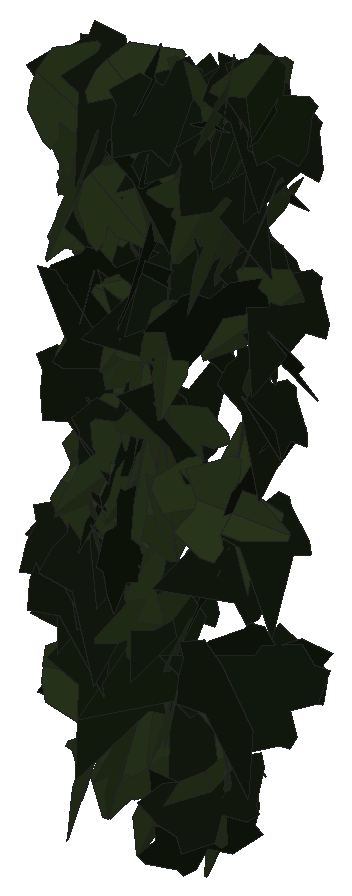
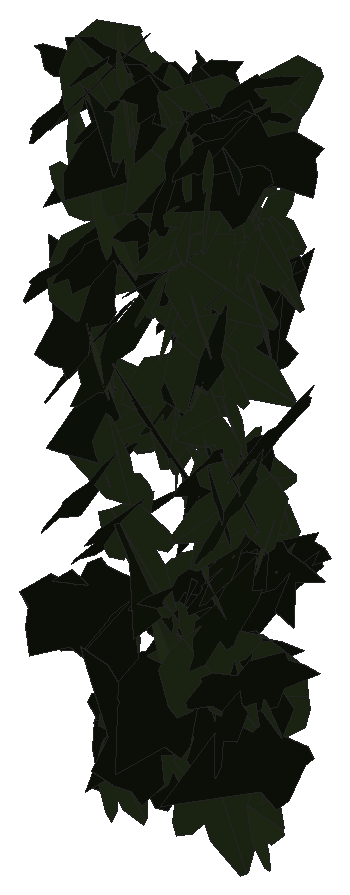
# SketchUp Ruby script. Lengths in inches.
U = 1.inch
M = Sketchup.active_model
def pt(a) = Geom::Point3d.new(a.map { |v| v * U })
def face(e, loops, mat)
  f = e.add_face(loops[0].map { |a| pt(a) })
  loops[1..].each { |l| e.add_face(l.map { |a| pt(a) }).erase! }
  f.material = f.back_material = mat if mat
  f
end
# faces: each face lists its corners as indices into pts; further lists are holes
def faces(e, pts, list, mat = nil) = list.each { |f| face(e, (f[0].is_a?(Array) ? f : [f]).map { |l| l.map { |i| pts[i] } }, mat) }
# xy, xz, yz: faces in a plane at the given z, y or x. An outline is a flat list of corners, or four numbers for a rectangle; further outlines are holes
def ring(l) = l.size == 4 ? [[l[0], l[1]], [l[2], l[1]], [l[2], l[3]], [l[0], l[3]]] : l.each_slice(2).to_a
def flat(e, list, mat, &to3) = list.each { |f| face(e, (f[0].is_a?(Array) ? f : [f]).map { |l| ring(l).map { |u, v| to3.(u, v) } }, mat) }
def xy(e, z, list, mat = nil) = flat(e, list, mat) { |x, y| [x, y, z] }
def xz(e, y, list, mat = nil) = flat(e, list, mat) { |x, z| [x, y, z] }
def yz(e, x, list, mat = nil) = flat(e, list, mat) { |y, z| [x, y, z] }
def lines(e, pts, list) = list.each { |a, b| e.add_line(pt(pts[a]), pt(pts[b])) }
# prism: a flat outline (further loops are holes) pulled along v
def prism(e, loops, v, mat = nil)
  f = face(e, loops, mat); d = Geom::Vector3d.new(v.map { |x| x * U })
  f.pushpull(f.normal.samedirection?(d) ? d.length : -d.length)
end
def box(e, o, s, mat = nil) = prism(e, [[o, [o[0] + s[0], o[1], o[2]], [o[0] + s[0], o[1] + s[1], o[2]], [o[0], o[1] + s[1], o[2]]]], [0, 0, s[2]], mat)
def at(x, y, z, deg = 0) = Geom::Transformation.translation(pt([x, y, z])) * Geom::Transformation.rotation(ORIGIN, Z_AXIS, deg.degrees)
def axes(o, x, y, z) = Geom::Transformation.new([*x, 0, *y, 0, *z, 0, *pt(o).to_a, 1])
def part(name) = M.definitions.add(name)
# library, detail: a bought-in or finely detailed component or shape, given as its bounding box
def library(name, o, s) = part(name).tap { |d| box(d.entities, o, s) }
def detail(e, o, s) = box(e.add_group.entities, o, s)
def put(e, d, t, mat = nil) = e.add_instance(d, t).tap { |i| i.material = mat if mat }
def group(e, t, mat = nil) = e.add_group.tap { |g| g.transformation = t; g.material = mat if mat }.entities
root = M.entities
M.materials.add("efeu1").color = [18, 25, 13]
M.materials.add("efeu2").color = [43, 57, 29]
c1 = part("ivyleaf_10")
p = [[0,0.5,-0.03],[-0.0625,2.02,-0.43],[-0.19,2.01,-0.46],[-0.54,1.05,-0.29],[-0.52,0.625,-0.18],[-0.83,0.76,-0.28],
  [-1.16,0.64,-0.33],[-1.15,0.33,-0.24],[-0.77,-0.39,0.02],[-0.3,-0.51,0.16],[0.04,-0.48,0.23],[-0.02,2.01,-0.4375],
  [-0.06,2.01,-0.43],[0.04,-0.49,0.23],[0.67,-0.49,0.14],[1.38,0.36,-0.2],[1.375,0.51,-0.24],[0.81,0.65,-0.19],
  [0.62,0.59,-0.15],[0.6,1.09,-0.28],[0.5,1.23,-0.31]]
faces(c1.entities,p,[[0,1,2,3,4,5,6,7,8,9,10],[11,12,0,13,14,15,16,17,18,19,20]],"efeu2")
c2 = part("ivyleaf_9")
p = [[1.54,2.16,1.25],[1.36,2.04,1.19],[-0.21,0.99,0.68],[-0.71,1.11,0.82],[-0.85,0.86,0.67],[-0.8,0.17,0.21],
  [-0.9,-0.01,0.1],[-0.67,-0.16,-0.02],[-0.08,-0.08,-0.05],[-0.03,-0.6,-0.4],[0.65,-0.88,-0.66],[0.83,-0.6,-0.49],
  [1.29,-0.42,-0.43],[1.8125,-0.07,-0.26],[1.21,0.44,0.15]]
faces(c2.entities,p,[[0,1,2,3,4,5,6,7,8,9,10,11,12,13,14]],"efeu1")
put(root,c1,axes([27.62,223.03,222.28],[-0.11697,0.34402,0.34346],[-0.14609,0.31206,-0.36232],[-0.46365,-0.18512,0.02751]))
put(root,c1,axes([27.55,223.54,221.27],[0.03739,0.32333,-0.37955],[-0.06683,-0.37393,-0.32513],[-0.4941,0.07505,0.01526]))
put(root,c2,axes([27.52,223.98,215.93],[-0.21987,-0.44229,-0.07768],[0.02759,0.07302,-0.49387],[0.44821,-0.22146,-0.0077]))
put(root,c2,axes([27.39,223.53,218.86],[0.19306,-0.44712,-0.11317],[-0.0519,0.10084,-0.48697],[0.45829,0.19978,-0.00747]))
put(root,c2,axes([27.375,223.71,222.54],[-0.12128,-0.22527,-0.42959],[0.20632,0.37681,-0.25583],[0.43901,-0.23932,0.00156]))
put(root,c1,axes([27.28,223.71,221.07],[0.31819,-0.13145,-0.3626],[0.33005,-0.15042,0.34416],[-0.19956,-0.45836,-0.00895]))
put(root,c2,axes([27.39,223.49,215.01],[0.39095,0.21573,0.22498],[0.19849,0.10596,-0.44651],[-0.24033,0.43845,-0.00279]))
put(root,c1,axes([27.84,223.37,221.11],[0.34552,-0.1496,-0.32899],[-0.30547,0.12234,-0.37646],[0.19313,0.46114,-0.00686]))
put(root,c1,axes([27.52,223.64,214.11],[0.14054,-0.2724,0.39503],[0.22811,-0.32421,-0.30472],[0.42215,0.26587,0.03314]))
put(root,c1,axes([27.64,222.8125,222.76],[-0.005,0.38256,0.3219],[-0.00797,0.32182,-0.38258],[-0.49991,-0.00896,0.00287]))
put(root,c1,axes([27.61,223.36,217.67],[-0.28743,0.38171,-0.14724],[0.09836,-0.11019,-0.47768],[-0.39712,-0.30357,-0.01175]))
put(root,c2,axes([27.59,224.21,216.52],[0.36352,-0.31201,-0.14321],[0.1085,-0.09347,0.47905],[-0.32571,-0.37936,-0.00025]))
put(root,c2,axes([27.48,224.22,218.04],[0.12998,-0.39691,0.2749],[0.08647,-0.26095,-0.41765],[0.475,0.15611,0.0008]))
put(root,c1,axes([27.72,223.53,220.59],[0.31674,-0.38292,0.0552],[0.03701,-0.04102,-0.49694],[0.38511,0.31889,0.00235]))
put(root,c1,axes([28.05,223.75,219.66],[-0.20976,-0.14352,0.43059],[-0.29469,-0.3177,-0.24945],[0.34519,-0.35843,0.04869]))
put(root,c1,axes([27.58,223.7,218.11],[-0.21848,-0.17739,-0.41328],[0.3336,0.24423,-0.28118],[0.30163,-0.3986,0.01163]))
put(root,c1,axes([28.13,223.94,220.74],[-0.18668,-0.15912,0.4357],[-0.3514,-0.25805,-0.2448],[0.30277,-0.39761,-0.01549]))
put(root,c2,axes([27.63,223.23,216.64],[0.10242,-0.48129,-0.08872],[-0.01362,0.08781,-0.49204],[0.48921,0.10321,0.00488]))
put(root,c2,axes([27.67,223.36,217.09],[-0.06574,-0.46362,-0.1753],[0.04884,0.16992,-0.4677],[0.49325,-0.07861,0.02294]))
put(root,c2,axes([27.88,223.4,217.13],[-0.41801,-0.22827,-0.15218],[0.13083,0.07792,-0.47625],[0.24114,-0.43797,-0.00541]))
put(root,c2,axes([27.73,223.96,222.53],[-0.05898,-0.49471,-0.04221],[0.00416,0.04202,-0.49821],[0.49649,-0.05912,-0.00084]))
put(root,c1,axes([28.03,223.74,214.28],[-0.35348,-0.31104,0.16825],[-0.12574,-0.11179,-0.47084],[0.33052,-0.37518,0.00081]))
put(root,c2,axes([28.01,223.47,219.51],[0.12075,0.10301,0.47414],[-0.41615,-0.22923,0.15578],[0.24947,-0.43225,0.03037]))
put(root,c1,axes([27.57,223.14,215.31],[0.07465,-0.03766,0.49296],[0.36183,0.3439,-0.02852],[-0.33691,0.36099,0.0786]))
put(root,c1,axes([28.01,223.72,219.44],[0.36886,-0.26696,-0.20658],[-0.15325,0.1402,-0.45482],[0.30076,0.39884,0.0216]))
put(root,c1,axes([28.14,223.94,215.92],[-0.26186,-0.28086,0.32023],[-0.20948,-0.24239,-0.38388],[0.37088,-0.33521,0.00928]))
put(root,c1,axes([27.87,223.52,217.96],[-0.30277,-0.31032,-0.24907],[0.16484,0.18704,-0.43341],[0.36216,-0.34456,-0.01096]))
put(root,c1,axes([27.97,223.77,222.11],[0.08898,-0.40796,-0.27505],[-0.00208,0.27919,-0.41478],[0.49201,0.07496,0.04799]))
put(root,c1,axes([28.1,222.8,221.63],[0.08549,-0.10265,0.48182],[-0.27531,0.39558,0.13312],[-0.40853,-0.28806,0.01111]))
put(root,c1,axes([27.99,224.23,219.9],[-0.0738,-0.34521,0.35409],[0.03484,-0.36076,-0.34444],[0.49329,-0.02617,0.0773]))
put(root,c1,axes([27.98,223.55,217.92],[0.00771,-0.10468,0.48886],[0.06083,-0.48509,-0.10483],[0.49623,0.06109,0.00526]))
put(root,c2,axes([27.99,223.62,218.31],[-0.37986,0.0896,-0.31253],[0.29876,-0.09341,-0.3899],[-0.12826,-0.48296,0.01743]))
put(root,c1,axes([27.875,223.4,215.36],[0.45063,-0.18147,0.11831],[0.11229,-0.03787,-0.48576],[0.18526,0.46437,0.00663]))
put(root,c2,axes([27.68,223.72,222.2],[0.46793,0.03531,0.17261],[0.17246,0.00852,-0.46924],[-0.03608,0.49868,-0.0042]))
put(root,c2,axes([27.86,223.7,218.39],[0.1023,-0.38206,-0.30589],[-0.07716,0.296,-0.39551],[0.4833,0.12813,0.0016]))
put(root,c2,axes([27.99,223.67,222.72],[-0.19475,-0.4507,0.09457],[-0.04612,-0.08308,-0.49089],[0.4582,-0.19992,-0.00921]))
put(root,c1,axes([28.11,223.86,219.4],[-0.21673,0.45039,-0.01323],[-0.0175,0.00625,0.49965],[0.45025,0.21704,0.01306]))
put(root,c2,axes([27.72,223.75,217.34],[0.25034,-0.38927,0.18921],[0.09983,-0.16075,-0.46281],[0.42115,0.26949,-0.00276]))
put(root,c1,axes([28.18,223.52,221.34],[-0.44166,0.18134,0.1485],[-0.15019,0.02426,-0.47629],[-0.17995,-0.46532,0.03305]))
put(root,c1,axes([27.74,223.22,217.58],[-0.24226,-0.07667,-0.43062],[0.43712,-0.05974,-0.23528],[-0.01537,-0.49046,0.09598]))
put(root,c2,axes([27.96,223.46,216.8],[-0.12437,-0.48404,-0.01536],[0.00412,0.01481,-0.49976],[0.48427,-0.12444,0.00031]))
put(root,c1,axes([28.18,223.65,221.83],[-0.41565,-0.2692,0.06904],[-0.0556,-0.04116,-0.49519],[0.27229,-0.41933,0.00428]))
put(root,c2,axes([27.85,223.7,220.63],[0.0261,-0.45423,0.20736],[0.08984,-0.19998,-0.44937],[0.49117,0.06072,0.07118]))
put(root,c2,axes([28.02,223.84,218.33],[-0.25037,0.05128,-0.42975],[0.40144,-0.15804,-0.25273],[-0.16175,-0.47159,0.03797]))
put(root,c2,axes([28.38,223.18,222.45],[-0.12737,0.37464,0.30566],[-0.09861,0.28931,-0.3957],[-0.47334,-0.16108,0.00019]))
put(root,c2,axes([28.29,223.08,220.58],[0.18669,0.29547,-0.35756],[-0.1922,-0.3015,-0.3495],[-0.42214,0.26794,0.001]))
put(root,c2,axes([27.8,223.96,215.09],[0.11093,-0.14238,0.46629],[0.25693,-0.38934,-0.18001],[0.41435,0.27954,-0.01321]))
put(root,c1,axes([27.84,224.01,219.05],[0.30038,-0.01739,0.39933],[0.39814,-0.03126,-0.30084],[0.03543,0.49872,-0.00493]))
put(root,c1,axes([28.05,223.85,216.95],[0.3384,-0.27129,0.24878],[0.18203,-0.17038,-0.4334],[0.31992,0.38389,-0.01654]))
put(root,c1,axes([28.05,223.49,222.69],[0.17794,0.36963,0.28585],[0.12651,0.25634,-0.41023],[-0.44981,0.21832,-0.0023]))
put(root,c2,axes([27.95,224.21,219.58],[-0.01471,-0.17478,0.46822],[0.22119,-0.42233,-0.1507],[0.44817,0.2027,0.08975]))
put(root,c1,axes([28.17,223.82,220.23],[0.26962,-0.38475,0.17109],[0.0923,-0.14422,-0.46977],[0.41083,0.2849,-0.00674]))
put(root,c1,axes([28.28,223.67,222.11],[0.03232,-0.4975,0.03807],[-0.00134,-0.03823,-0.49853],[0.49895,0.03212,-0.00381]))
put(root,c1,axes([28.1,223.32,214.5],[-0.22813,-0.33558,0.29213],[0.15259,0.24937,0.40562],[-0.41794,0.27422,-0.01137]))
put(root,c1,axes([28.21,222.98,221.62],[0.01468,0.41147,0.28368],[-0.01259,0.28402,-0.41131],[-0.49963,0.00493,0.0187]))
put(root,c2,axes([28.3,223.36,215.6875],[-0.32546,-0.37925,-0.01575],[0.01249,0.01004,-0.49974],[0.37937,-0.32569,0.00294]))
put(root,c1,axes([28.05,223.76,221.28],[-0.11996,-0.27216,-0.40192],[0.36792,0.21907,-0.25816],[0.31662,-0.35768,0.14771]))
put(root,c1,axes([28.31,223.27,214.72],[0.14879,-0.47599,0.03598],[0.01557,-0.03283,-0.49868],[0.47709,0.14952,0.00505]))
put(root,c1,axes([28.21,223.78,217.95],[-0.01906,-0.15372,0.4754],[0.17014,-0.44931,-0.13847],[0.46978,0.15649,0.06944]))
put(root,c1,axes([28.46,223.55,220.16],[-0.08133,-0.33567,0.36154],[0.01254,-0.36771,-0.33857],[0.49318,-0.046,0.06823]))
put(root,c2,axes([28.24,224.33,222.02],[0.06537,-0.16936,-0.46588],[0.36077,-0.30601,0.16187],[-0.33996,-0.35731,0.0822]))
put(root,c1,axes([28.49,224.12,222.1],[0.14529,0.365,-0.3093],[-0.18632,-0.25456,-0.38792],[-0.44065,0.22798,0.06204]))
put(root,c2,axes([28.52,222.86,217.56],[0.14629,-0.12413,-0.46172],[-0.34282,0.30934,-0.19178],[0.33328,0.37269,0.0054]))
put(root,c1,axes([28.42,223.27,217.56],[0.41634,-0.26982,0.06209],[-0.04805,0.04001,0.49608],[-0.27267,-0.41904,0.00738]))
put(root,c2,axes([28.38,223.33,220.16],[0.02319,0.32753,0.37708],[-0.06538,-0.37224,0.32735],[0.49516,-0.06449,0.02556]))
put(root,c1,axes([28.4375,223.96,221.5],[-0.40616,0.2468,-0.15531],[0.11697,-0.10605,-0.47442],[-0.26712,-0.42171,0.02841]))
put(root,c1,axes([28.66,223.53,219.875],[0.05111,0.31385,0.38586],[-0.11313,-0.37039,0.31625],[0.48435,-0.11963,0.03315]))
put(root,c2,axes([28.51,223.87,216.66],[-0.16027,-0.4554,0.13009],[-0.01248,-0.13322,-0.48176],[0.47345,-0.15767,0.03133]))
put(root,c1,axes([28.52,223.83,220.27],[-0.13869,0.34731,-0.33188],[0.05869,-0.3306,-0.37049],[-0.47678,-0.14172,0.05093]))
put(root,c1,axes([28.71,223.23,216.47],[-0.18531,-0.46341,-0.03026],[0.01179,0.02788,-0.49908],[0.46424,-0.18568,0.0006]))
put(root,c2,axes([28.38,223.51,221.64],[0.07832,-0.37754,0.31833],[0.18172,-0.27765,-0.37401],[0.45918,0.17428,0.09372]))
put(root,c2,axes([28.75,223.55,219.98],[-0.13321,-0.16462,0.45294],[-0.22309,-0.39548,-0.20934],[0.42719,-0.25786,0.03191]))
put(root,c2,axes([28.65,223.8,218.22],[-0.29473,0.35444,0.19366],[0.11972,-0.1523,0.46095],[0.38575,0.31808,0.0049]))
put(root,c1,axes([28.5,223.22,216.74],[0.33724,-0.29747,-0.21859],[0.18454,-0.12057,0.44879],[-0.31971,-0.38337,0.02847]))
put(root,c1,axes([28.99,223.62,222.63],[0.22307,-0.16282,-0.41681],[-0.33807,0.24381,-0.27617],[0.29317,0.40503,-0.00131]))
put(root,c2,axes([28.7,223.92,220.47],[-0.24091,-0.3459,0.26891],[0.01297,-0.31238,-0.39019],[0.43794,-0.18102,0.15948]))
put(root,c2,axes([29.02,223.46,216.02],[-0.45566,-0.14033,0.15059],[-0.14433,-0.04299,-0.47678],[0.14676,-0.47797,-0.00133]))
put(root,c1,axes([28.78,223.73,215.99],[0.22083,-0.43411,0.11305],[0.04869,-0.10207,-0.48704],[0.44594,0.22612,-0.0028]))
put(root,c2,axes([28.66,223.48,222.76],[-0.02232,-0.37082,-0.33465],[0.0284,0.3335,-0.37144],[0.49869,-0.03559,0.00618]))
put(root,c1,axes([28.85,223.3,215.49],[0.35183,-0.35027,-0.0594],[-0.03482,0.0492,-0.49635],[0.35356,0.3534,0.01023]))
put(root,c1,axes([28.93,223.3125,214.46],[-0.07787,-0.4604,0.17879],[-0.03356,-0.17565,-0.46693],[0.49276,-0.08471,-0.00354]))
put(root,c1,axes([28.91,223.31,218.85],[-0.45836,-0.19892,-0.0183],[0.01677,0.00731,-0.49967],[0.19905,-0.45867,-0.00003]))
put(root,c2,axes([28.85,223.57,218.65],[0.25522,-0.41434,-0.11484],[0.06246,-0.0964,0.48663],[-0.4254,-0.26274,0.00256]))
put(root,c2,axes([28.71,223.71,215.22],[0.49418,0.06213,-0.04387],[-0.04429,0.00066,-0.49803],[-0.06183,0.49612,0.00616]))
put(root,c2,axes([29.17,223.66,222.61],[-0.49917,0.00222,0.02868],[-0.02868,0.00063,-0.49918],[-0.00225,-0.49999,-0.00051]))
put(root,c2,axes([29.12,223.52,216.56],[-0.04063,0.31279,0.38796],[-0.03597,0.38639,-0.31529],[-0.49705,-0.05353,-0.0089]))
put(root,c1,axes([29.17,223.875,217.17],[0.40711,-0.09193,-0.27533],[-0.26163,0.08922,-0.41664],[0.12574,0.48331,0.02454]))
put(root,c1,axes([28.97,223.22,220.09],[0.04643,0.46584,-0.17561],[-0.02949,-0.17349,-0.46801],[-0.49697,0.05382,0.01137]))
put(root,c1,axes([29.18,223.67,221.61],[-0.24028,-0.39194,0.1966],[-0.1119,-0.16195,-0.45962],[0.42396,-0.26487,-0.00989]))
put(root,c1,axes([29.08,223.85,222.27],[0.02483,-0.49029,-0.09487],[-0.00237,0.09487,-0.49091],[0.49938,0.02483,0.00239]))
put(root,c1,axes([29.25,222.79,217.9],[-0.08421,0.28491,-0.40217],[-0.17894,0.36248,0.29426],[0.45923,0.19348,0.04091]))
put(root,c2,axes([28.9375,223.65,214.36],[0.17031,0.46457,0.07187],[-0.03704,-0.06295,0.49464],[0.46864,-0.17381,0.01297]))
put(root,c1,axes([29.1875,223.36,214.68],[0.47042,-0.07945,0.14963],[-0.14707,0.02766,0.47708],[-0.08409,-0.49287,0.00266]))
put(root,c2,axes([29,223.74,222.16],[0.48917,0.07467,0.0717],[0.0689,0.02363,-0.49467],[-0.07726,0.49383,0.01283]))
put(root,c1,axes([29.35,223.625,222.91],[0.11977,-0.43587,-0.21372],[-0.05838,0.20559,-0.45202],[0.48192,0.13323,-0.00164]))
put(root,c2,axes([29.35,223.33,213.73],[0.25233,0.11004,0.4174],[-0.38039,-0.17185,0.27526],[0.20404,-0.45646,-0.00301]))
put(root,c2,axes([29.42,224.03,217],[-0.25635,-0.18069,0.3894],[-0.14918,-0.38779,-0.27814],[0.40253,-0.25879,0.14491]))
put(root,c1,axes([29.26,223.83,217.59],[0.49659,-0.05214,-0.02598],[0.02584,-0.0027,0.49932],[-0.05221,-0.49727,0.00001]))
put(root,c1,axes([29.375,223.93,221.18],[0.13877,-0.46792,0.10859],[0.01671,-0.10826,-0.48785],[0.48007,0.13903,-0.01441]))
put(root,c1,axes([29.35,223.86,214.22],[0.09593,-0.4388,0.21966],[0.07228,-0.20874,-0.44855],[0.48536,0.11782,0.02339]))
put(root,c2,axes([29.5625,223.11,220.63],[0.03503,0.44543,-0.22442],[-0.03925,-0.22181,-0.44638],[-0.49722,0.04889,0.01943]))
put(root,c2,axes([29.68,223.62,222.37],[-0.09405,0.38093,0.30992],[-0.10218,0.29347,-0.39171],[-0.48033,-0.13701,0.02265]))
put(root,c1,axes([29.26,222.76,218.11],[-0.04967,-0.0607,-0.49381],[0.31401,0.38111,-0.07844],[0.38592,-0.31791,0.00026]))
put(root,c2,axes([29.29,224.03,220.73],[0.05846,-0.4666,-0.1699],[-0.01398,0.16946,-0.4702],[0.49637,0.05973,0.00677]))
put(root,c2,axes([29.6875,223.12,214.39],[-0.3516,-0.33181,0.12759],[0.09395,0.08635,0.48344],[-0.34286,0.36393,0.00163]))
put(root,c1,axes([29.54,224.1,222.98],[-0.05143,-0.44616,0.21977],[0.02359,-0.22288,-0.44695],[0.49679,-0.0356,0.04397]))
put(root,c2,axes([29.18,224.0625,219.34],[0.18958,-0.39552,0.24006],[0.16091,-0.18687,-0.43496],[0.43378,0.24217,0.05643]))
put(root,c1,axes([29.54,223.13,214.66],[-0.18057,-0.44737,-0.13136],[0.05692,0.11867,-0.48237],[0.46277,-0.18916,0.00807]))
put(root,c2,axes([29.4,223.54,222.21],[0.12444,-0.43363,-0.21559],[-0.03209,0.21472,-0.45041],[0.4832,0.12593,0.02561]))
put(root,c1,axes([29.49,224,219.46],[0.26413,-0.35613,0.23109],[0.15922,-0.16921,-0.44274],[0.39355,0.30747,0.02402]))
put(root,c2,axes([29.4,224.14,222.7],[0.04167,-0.47822,0.13989],[0.04944,-0.13572,-0.47868],[0.4958,0.05373,0.03597]))
put(root,c1,axes([29.55,223.36,221.47],[0.1522,-0.36001,0.31181],[0.1215,-0.28717,-0.39086],[0.46051,0.19475,0.00006]))
put(root,c1,axes([29.39,223.53,214.8],[-0.09312,0.05382,0.4883],[0.40833,-0.26783,0.10739],[0.27312,0.41877,0.00593]))
put(root,c1,axes([29.77,224.06,220.27],[-0.03796,-0.18628,0.46245],[-0.07182,-0.45691,-0.18994],[0.49336,-0.08085,0.00793]))
put(root,c2,axes([29.48,223.41,215.94],[0.13667,-0.48063,-0.01777],[-0.00326,0.01755,-0.49968],[0.48095,0.1367,0.00166]))
put(root,c2,axes([29.84,223.97,222.87],[-0.46169,-0.19145,0.01355],[-0.01121,-0.00833,-0.4998],[0.1916,-0.46182,0.0034]))
put(root,c2,axes([29.875,223.83,216.11],[0.11541,0.2479,-0.4186],[-0.15881,-0.38745,-0.27324],[-0.45985,0.19603,-0.01069]))
put(root,c2,axes([29.5625,224.05,217.65],[0.06451,-0.49323,0.0506],[0.00918,-0.04983,-0.49743],[0.49574,0.06511,0.00262]))
put(root,c2,axes([29.77,223.31,218.06],[0.08849,0.17779,0.45887],[0.13381,0.43997,-0.19627],[-0.47356,0.15754,0.03029]))
put(root,c2,axes([30.14,223.7,215.55],[-0.15192,0.04772,0.47397],[-0.47634,-0.0205,-0.15061],[0.00506,-0.4973,0.05169]))
put(root,c1,axes([29.625,224,221.17],[0.05354,-0.44958,-0.21217],[0.11642,-0.19612,0.44495],[-0.4833,-0.09705,0.08368]))
put(root,c2,axes([29.72,224.31,222.45],[-0.08429,-0.43731,0.22728],[-0.04768,-0.22226,-0.44534],[0.49053,-0.09675,-0.00424]))
put(root,c1,axes([29.49,223.03,218.15],[0.09531,0.1066,0.47912],[0.34994,0.32747,-0.14248],[-0.34417,0.36249,-0.01218]))
put(root,c2,axes([29.72,224.28,220.46],[-0.0944,-0.47089,0.13911],[-0.02559,-0.13675,-0.48025],[0.49034,-0.09779,0.00172]))
put(root,c2,axes([29.46,224.17,219.71],[0.39348,-0.04022,-0.30586],[0.3027,-0.04528,0.39537],[-0.05951,-0.49632,-0.01129]))
put(root,c2,axes([29.66,224.04,219.19],[0.03761,-0.45993,0.19247],[0.01068,-0.19223,-0.46145],[0.49847,0.03882,-0.00464]))
